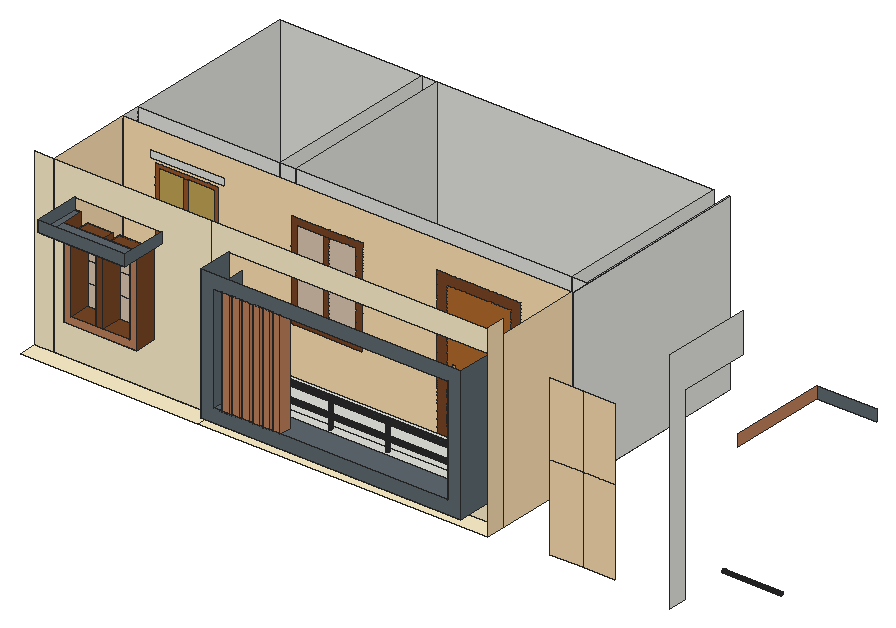
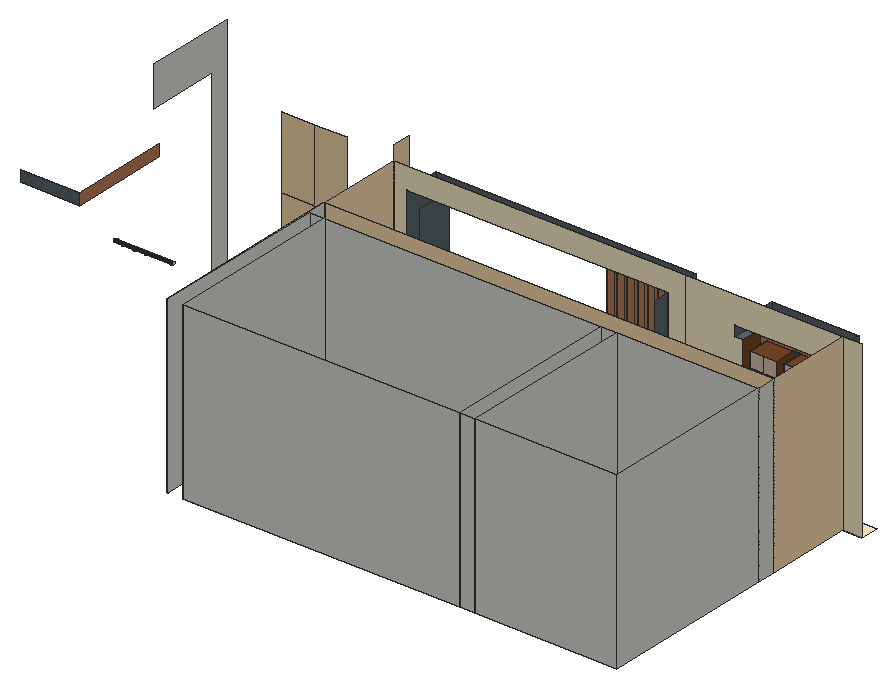
# SketchUp Ruby script. Lengths in inches.
U = 1.inch
M = Sketchup.active_model
def pt(a) = Geom::Point3d.new(a.map { |v| v * U })
def face(e, loops, mat)
  f = e.add_face(loops[0].map { |a| pt(a) })
  loops[1..].each { |l| e.add_face(l.map { |a| pt(a) }).erase! }
  f.material = f.back_material = mat if mat
  f
end
# faces: each face lists its corners as indices into pts; further lists are holes
def faces(e, pts, list, mat = nil) = list.each { |f| face(e, (f[0].is_a?(Array) ? f : [f]).map { |l| l.map { |i| pts[i] } }, mat) }
# xy, xz, yz: faces in a plane at the given z, y or x. An outline is a flat list of corners, or four numbers for a rectangle; further outlines are holes
def ring(l) = l.size == 4 ? [[l[0], l[1]], [l[2], l[1]], [l[2], l[3]], [l[0], l[3]]] : l.each_slice(2).to_a
def flat(e, list, mat, &to3) = list.each { |f| face(e, (f[0].is_a?(Array) ? f : [f]).map { |l| ring(l).map { |u, v| to3.(u, v) } }, mat) }
def xy(e, z, list, mat = nil) = flat(e, list, mat) { |x, y| [x, y, z] }
def xz(e, y, list, mat = nil) = flat(e, list, mat) { |x, z| [x, y, z] }
def yz(e, x, list, mat = nil) = flat(e, list, mat) { |y, z| [x, y, z] }
def lines(e, pts, list) = list.each { |a, b| e.add_line(pt(pts[a]), pt(pts[b])) }
# prism: a flat outline (further loops are holes) pulled along v
def prism(e, loops, v, mat = nil)
  f = face(e, loops, mat); d = Geom::Vector3d.new(v.map { |x| x * U })
  f.pushpull(f.normal.samedirection?(d) ? d.length : -d.length)
end
def box(e, o, s, mat = nil) = prism(e, [[o, [o[0] + s[0], o[1], o[2]], [o[0] + s[0], o[1] + s[1], o[2]], [o[0], o[1] + s[1], o[2]]]], [0, 0, s[2]], mat)
def at(x, y, z, deg = 0) = Geom::Transformation.translation(pt([x, y, z])) * Geom::Transformation.rotation(ORIGIN, Z_AXIS, deg.degrees)
def axes(o, x, y, z) = Geom::Transformation.new([*x, 0, *y, 0, *z, 0, *pt(o).to_a, 1])
def part(name) = M.definitions.add(name)
# library, detail: a bought-in or finely detailed component or shape, given as its bounding box
def library(name, o, s) = part(name).tap { |d| box(d.entities, o, s) }
def detail(e, o, s) = box(e.add_group.entities, o, s)
def put(e, d, t, mat = nil) = e.add_instance(d, t).tap { |i| i.material = mat if mat }
def group(e, t, mat = nil) = e.add_group.tap { |g| g.transformation = t; g.material = mat if mat }.entities
root = M.entities
M.materials.add("[Blinds Cloth Horizontal]").color = [192, 163, 85]
M.materials.add("[Color C01]").color = [221, 199, 177]
M.materials.add("[Color D01]").color = [255, 242, 204]
M.materials.add("[Formica Beige]").color = [255, 225, 180]
M.materials.add("[Formica Beige]1").color = [247, 219, 174]
M.materials.add("[Formica Laminate Dark]").color = [50, 53, 60]
M.materials.add("[Formica Speckled Grey]").color = [94, 105, 111]
M.materials.add("[Wood Bamboo]").color = [177, 105, 43]
M.materials.add("[Wood Cherry Original]").color = [152, 86, 42]
M.materials.add("[Wood Floor Light]").color = [204, 176, 127]
M.materials.add("[Wood Veneer 01]").color = [120, 70, 37]
M.materials.add("[Wood Veneer 02]").color = [190, 128, 91]
xy(root,536.125,[[47.7,166.1,1198.27,388.54],[47.7,388.54,1201.41,436.38],[1201.41,388.54,1201.79,436.38],[47.7,436.38,412.34,890.39],[412.34,436.38,451.3125,890.39],
  [451.3125,436.38,1159.05,890.39],[1198.27,436.38,1198.27,890.39,1201.41,436.38],[1201.41,436.38,1198.27,890.39,1201.41,890.39],[1201.41,436.38,1201.79,890.39]])
xy(root,536.125,[[0,119.17,455.68,166.1],[455.68,119.17,1198.27,166.1]],"[Color D01]")
xy(root,585.01,[[497.875,73.92,1164.39,166.1]],"[Formica Speckled Grey]")
xy(root,588.32,[[1811.85,227.29,1812.63,227.4,1813.35,227.69,1813.97,228.17,1814.45,228.79,1814.75,229.52,1814.85,230.29,1814.75,231.07,1814.45,231.79,1813.97,232.41,1813.35,232.89,1812.63,233.19,1811.85,233.29,1811.08,233.19,1810.35,232.89,1809.73,232.41,1809.25,231.79,1808.96,231.07,1808.85,230.29,1808.96,229.52,1809.25,228.79,1809.73,228.17,1810.35,227.69,1811.08,227.4]])
xy(root,588.82,[[1840.85,227.29,1841.63,227.4,1842.35,227.69,1842.97,228.17,1843.45,228.79,1843.75,229.52,1843.85,230.29,1843.75,231.07,1843.45,231.79,1842.97,232.41,1842.35,232.89,1841.63,233.19,1840.85,233.29,1840.08,233.19,1839.35,232.89,1838.73,232.41,1838.25,231.79,1837.96,231.07,1837.85,230.29,1837.96,229.52,1838.25,228.79,1838.73,228.17,1839.35,227.69,1840.08,227.4]])
xy(root,589.07,[[1780.92,227.29,1781.69,227.4,1782.42,227.69,1783.04,228.17,1783.51,228.79,1783.8125,229.52,1783.92,230.29,1783.8125,231.07,1783.51,231.79,1783.04,232.41,1782.42,232.89,1781.69,233.19,1780.92,233.29,1780.14,233.19,1779.42,232.89,1778.79,232.41,1778.32,231.79,1778.02,231.07,1777.92,230.29,1778.02,229.52,1778.32,228.79,1778.79,228.17,1779.42,227.69,1780.14,227.4]])
xy(root,591.76,[[1750.54,227.29,1751.32,227.4,1752.04,227.69,1752.66,228.17,1753.14,228.79,1753.4375,229.52,1753.54,230.29,1753.4375,231.07,1753.14,231.79,1752.66,232.41,1752.44,232.59,1748.65,232.59,1748.42,232.41,1747.94,231.79,1747.64,231.07,1747.54,230.29,1747.64,229.52,1747.94,228.79,1748.42,228.17,1749.04,227.69,1749.76,227.4],[1748.65,232.59,1752.44,232.59,1752.04,232.89,1751.32,233.19,1750.54,233.29,1749.76,233.19,1749.04,232.89]])
xy(root,592.19,[[1855.17,227.29,1855.94,227.4,1856.67,227.69,1857.29,228.17,1857.76,228.79,1858.0625,229.52,1858.17,230.29,1858.0625,231.07,1857.76,231.79,1857.29,232.41,1856.67,232.89,1855.94,233.19,1855.17,233.29,1854.39,233.19,1853.67,232.89,1853.04,232.41,1852.57,231.79,1852.27,231.07,1852.17,230.29,1852.27,229.52,1852.57,228.79,1853.04,228.17,1853.67,227.69,1854.39,227.4]])
xy(root,593.51,[[1722.85,227.29,1723.63,227.4,1724.35,227.69,1724.97,228.17,1725.45,228.79,1725.75,229.52,1725.85,230.29,1725.75,231.07,1725.45,231.79,1725.2,232.12,1720.5,232.12,1720.25,231.79,1719.96,231.07,1719.85,230.29,1719.96,229.52,1720.25,228.79,1720.73,228.17,1721.35,227.69,1722.08,227.4],[1720.5,232.12,1725.2,232.12,1724.97,232.41,1724.35,232.89,1723.63,233.19,1722.85,233.29,1722.08,233.19,1721.35,232.89,1720.73,232.41]])
xy(root,618.32,[[553.83,73.92,572.52,104.16],[579.27,73.92,597.96,104.16],[604.77,73.92,623.46,104.16],[631.58,73.92,650.27,104.16],[657.77,73.92,676.46,104.16],
  [683.15,73.92,701.83,104.16],[[531.18,142.13,1131.08,166.1],[617.04,150.12,616.01,150.25,615.04,150.65,614.22,151.29,613.58,152.12,613.18,153.08,613.04,154.12,613.18,155.15,613.58,156.12,614.22,156.95,615.04,157.58,616.01,157.98,617.04,158.12,618.08,157.98,619.04,157.58,619.87,156.95,620.51,156.12,620.91,155.15,621.04,154.12,620.91,153.08,620.51,152.12,619.87,151.29,619.04,150.65,618.08,150.25],[913.79,150.12,912.76,150.25,911.79,150.65,910.97,151.29,910.33,152.12,909.93,153.08,909.79,154.12,909.93,155.15,910.33,156.12,910.97,156.95,911.79,157.58,912.76,157.98,913.79,158.12,914.83,157.98,915.79,157.58,916.62,156.95,917.26,156.12,917.66,155.15,917.79,154.12,917.66,153.08,917.26,152.12,916.62,151.29,915.79,150.65,914.83,150.25],[767.42,150.12,766.38,150.25,765.42,150.65,764.59,151.29,763.95,152.12,763.56,153.08,763.42,154.12,763.56,155.15,763.95,156.12,764.59,156.95,765.42,157.58,766.38,157.98,767.42,158.12,768.45,157.98,769.42,157.58,770.25,156.95,770.88,156.12,771.28,155.15,771.42,154.12,771.28,153.08,770.88,152.12,770.25,151.29,769.42,150.65,768.45,150.25],[1075.98,150.12,1074.95,150.25,1073.98,150.65,1073.15,151.29,1072.52,152.12,1072.12,153.08,1071.98,154.12,1072.12,155.15,1072.52,156.12,1073.15,156.95,1073.98,157.58,1074.95,157.98,1075.98,158.12,1077.02,157.98,1077.98,157.58,1078.81,156.95,1079.45,156.12,1079.84,155.15,1079.98,154.12,1079.84,153.08,1079.45,152.12,1078.81,151.29,1077.98,150.65,1077.02,150.25]],[617.04,150.12,616.01,150.25,615.04,150.65,614.22,151.29,613.58,152.12,613.18,153.08,613.04,154.12,613.18,155.15,613.58,156.12,614.22,156.95,615.04,157.58,616.01,157.98,617.04,158.12,618.08,157.98,619.04,157.58,619.87,156.95,620.51,156.12,620.91,155.15,621.04,154.12,620.91,153.08,620.51,152.12,619.87,151.29,619.04,150.65,618.08,150.25],[767.42,150.12,766.38,150.25,765.42,150.65,764.59,151.29,763.95,152.12,763.56,153.08,763.42,154.12,763.56,155.15,763.95,156.12,764.59,156.95,765.42,157.58,766.38,157.98,767.42,158.12,768.45,157.98,769.42,157.58,770.25,156.95,770.88,156.12,771.28,155.15,771.42,154.12,771.28,153.08,770.88,152.12,770.25,151.29,769.42,150.65,768.45,150.25],[913.79,150.12,912.76,150.25,911.79,150.65,910.97,151.29,910.33,152.12,909.93,153.08,909.79,154.12,909.93,155.15,910.33,156.12,910.97,156.95,911.79,157.58,912.76,157.98,913.79,158.12,914.83,157.98,915.79,157.58,916.62,156.95,917.26,156.12,917.66,155.15,917.79,154.12,917.66,153.08,917.26,152.12,916.62,151.29,915.79,150.65,914.83,150.25],
  [1075.98,150.12,1074.95,150.25,1073.98,150.65,1073.15,151.29,1072.52,152.12,1072.12,153.08,1071.98,154.12,1072.12,155.15,1072.52,156.12,1073.15,156.95,1073.98,157.58,1074.95,157.98,1075.98,158.12,1077.02,157.98,1077.98,157.58,1078.81,156.95,1079.45,156.12,1079.84,155.15,1079.98,154.12,1079.84,153.08,1079.45,152.12,1078.81,151.29,1077.98,150.65,1077.02,150.25]])
xy(root,618.32,[[531.18,73.92,553.83,73.92,553.83,104.16,572.52,104.16,572.52,73.92,579.27,73.92,579.27,104.16,597.96,104.16,597.96,73.92,604.77,73.92,604.77,104.16,623.46,104.16,623.46,73.92,631.58,73.92,631.58,104.16,650.27,104.16,650.27,73.92,657.77,73.92,657.77,104.16,676.46,104.16,676.46,73.92,683.15,73.92,683.15,104.16,701.83,104.16,701.83,73.92,1131.08,73.92,1131.08,142.13,531.18,142.13]],"[Formica Speckled Grey]")
xy(root,654.42,[[117.05,111.6,304.55,166.1]],"[Wood Veneer 01]")
xy(root,672.82,[[135.45,111.6,199.22,166.1],[216.32,111.6,286.15,166.1]],"[Wood Veneer 01]")
xy(root,684.94,[[1075.98,150.12,1077.02,150.25,1077.98,150.65,1078.81,151.29,1079.45,152.12,1079.84,153.08,1079.98,154.12,1079.84,155.15,1079.45,156.12,1078.81,156.95,1077.98,157.58,1077.02,157.98,1075.98,158.12,1074.95,157.98,1073.98,157.58,1073.15,156.95,1072.52,156.12,1072.12,155.15,1071.98,154.12,1072.12,153.08,1072.52,152.12,1073.15,151.29,1073.98,150.65,1074.95,150.25]])
xy(root,686.94,[[913.79,150.12,914.83,150.25,915.79,150.65,916.62,151.29,917.26,152.12,917.66,153.08,917.79,154.12,917.66,155.15,917.26,156.12,916.62,156.95,915.79,157.58,914.83,157.98,913.79,158.12,912.76,157.98,911.79,157.58,910.97,156.95,910.33,156.12,909.93,155.15,909.79,154.12,909.93,153.08,910.33,152.12,910.97,151.29,911.79,150.65,912.76,150.25]])
xy(root,687.63,[[767.42,150.12,768.45,150.25,769.42,150.65,770.25,151.29,770.88,152.12,771.28,153.08,771.42,154.12,771.28,155.15,770.88,156.12,770.25,156.95,769.42,157.58,768.45,157.98,767.42,158.12,766.38,157.98,765.42,157.58,764.59,156.95,763.95,156.12,763.56,155.15,763.42,154.12,763.56,153.08,763.95,152.12,764.59,151.29,765.42,150.65,766.38,150.25]])
xy(root,688.88,[[617.04,150.12,618.08,150.25,619.04,150.65,619.87,151.29,620.51,152.12,620.91,153.08,621.04,154.12,620.91,155.15,620.51,156.12,619.87,156.95,619.04,157.58,618.08,157.98,617.04,158.12,616.01,157.98,615.04,157.58,614.22,156.95,613.58,156.12,613.18,155.15,613.04,154.12,613.18,153.08,613.58,152.12,614.22,151.29,615.04,150.65,616.01,150.25]])
xy(root,863.89,[[135.45,111.6,199.22,166.1],[216.32,111.6,286.15,166.1]],"[Wood Veneer 01]")
xy(root,882.3,[[100.99,47.54,117.05,166.1],[117.05,47.54,304.55,111.6],[304.55,47.54,326.11,166.1]],"[Formica Speckled Grey]")
xz(root,47.54,[[100.99,882.3,326.11,911.08]],"[Formica Speckled Grey]")
xz(root,73.92,[[[497.875,585.01,1164.39,925.7],[531.18,618.32,1131.08,892.39]]],"[Formica Speckled Grey]")
xz(root,73.92,[[553.83,618.32,572.52,892.39],[579.27,618.32,597.96,892.39],[604.77,618.32,623.46,892.39],[631.58,618.32,650.27,892.39],[657.77,618.32,676.46,892.39],
  [683.15,618.32,701.83,892.39]],"[Wood Veneer 02]")
xz(root,104.16,[[553.83,618.32,572.52,892.39],[579.27,618.32,597.96,892.39],[604.77,618.32,623.46,892.39],[631.58,618.32,650.27,892.39],[657.77,618.32,676.46,892.39],
  [683.15,618.32,701.83,892.39]],"[Wood Veneer 02]")
xz(root,111.6,[[199.22,672.82,216.32,863.89]],"[Wood Veneer 01]")
xz(root,111.6,[[[117.05,654.42,304.55,882.3],[135.45,672.82,286.15,863.89]]],"[Wood Veneer 02]")
xz(root,119.17,[[1358.02,552.78,1440.68,771.08],[1440.68,552.78,1523.35,771.08],[1358.02,771.08,1440.68,957.69],[1440.68,771.08,1523.35,957.69]],"[Formica Beige]1")
xz(root,166.1,[[135.45,672.82,167.34,726.34],[167.34,672.82,199.22,726.34],[216.32,672.82,251.23,726.34],[251.23,672.82,286.15,726.34],[135.45,726.34,167.34,779.86],
  [167.34,726.34,199.22,779.86],[216.32,726.34,251.23,779.86],[251.23,726.34,286.15,779.86],[135.45,779.86,167.34,824.51],[167.34,779.86,199.22,824.51],
  [216.32,779.86,251.23,824.51],[251.23,779.86,286.15,824.51],[135.45,824.51,167.34,863.89],[167.34,824.51,199.22,863.89],[216.32,824.51,251.23,863.89],
  [251.23,824.51,286.15,863.89]],"[Color C01]")
xz(root,166.1,[[0,536.125,47.7,980.9375],[[47.7,536.125,1198.27,980.3125],[497.875,585.01,1164.39,925.7],[117.05,654.42,117.05,882.3,100.99,882.3,100.99,911.08,326.11,911.08,326.11,882.3,304.55,882.3,304.55,654.42]]],"[Color D01]")
xz(root,388.54,[[1198.27,536.125,1201.41,980.3125],[1201.41,536.125,1201.79,980.3125]])
xz(root,388.54,[[142.36,701.45,201.48,892.8125],[216.65,701.45,279.66,892.8125]],"[Blinds Cloth Horizontal]")
xz(root,388.54,[[496.54,672.47,559.83,886.7],[575.8125,672.47,643.15,886.7]],"[Color C01]")
xz(root,388.54,[[[47.7,536.125,852.07,536.125,852.07,910.25,1068.07,910.25,1068.07,536.125,1198.27,536.125,1198.27,980.3125,47.7,980.3125],[477.9375,653.87,661.75,905.31],[130.08,689.16,291.95,905.1],[116.16,908.99,307.29,929.24]]],"[Formica Beige]")
xz(root,388.54,[[[877.66,561.71,1042.48,884.66],[890.09,623.15,901.34,708.15]]],"[Wood Bamboo]")
xz(root,388.54,[[[130.08,689.16,291.95,905.1],[142.36,701.45,279.66,892.8125]],[201.48,701.45,216.65,892.8125]],"[Wood Cherry Original]")
xz(root,388.54,[[890.09,623.15,901.34,708.15]],"[Wood Floor Light]")
xz(root,388.54,[[[852.07,536.125,1068.07,910.25],[877.66,561.71,1042.48,884.66]],[[477.9375,653.87,661.75,905.31],[496.54,672.47,643.15,886.7]],[559.83,672.47,575.8125,886.7]],"[Wood Veneer 01]")
xz(root,436.38,[[47.7,536.125,412.34,980.3125],[412.34,536.125,451.3125,980.3125],[451.3125,536.125,1159.05,980.3125],[1159.05,536.125,1198.27,980.3125]])
xz(root,528.45,[[1713.03,855.83,1866.15,885.01]],"[Formica Speckled Grey]")
xz(root,890.39,[[47.7,536.125,412.34,980.9375],[412.34,536.125,451.3125,980.9375],[451.3125,536.125,1159.05,980.9375],[1198.27,536.125,1201.41,980.3125],[1201.41,536.125,1201.79,536.125,1201.79,980.9375,1198.27,980.9375,1198.27,980.3125,1201.41,980.3125]])
yz(root,47.7,[[388.54,536.125,436.38,980.3125],[436.38,536.125,890.39,980.9375]])
yz(root,47.7,[[166.1,536.125,388.54,980.9375]],"[Formica Beige]")
yz(root,100.99,[[47.54,882.3,166.1,911.08]],"[Formica Speckled Grey]")
yz(root,117.05,[[111.6,654.42,166.1,882.3]],"[Wood Veneer 01]")
yz(root,135.45,[[111.6,672.82,166.1,863.89]],"[Wood Veneer 01]")
yz(root,199.22,[[111.6,672.82,166.1,863.89]],"[Wood Veneer 01]")
yz(root,216.32,[[111.6,672.82,166.1,863.89]],"[Wood Veneer 01]")
yz(root,286.15,[[111.6,672.82,166.1,863.89]],"[Wood Veneer 01]")
yz(root,304.55,[[111.6,654.42,166.1,882.3]],"[Wood Veneer 01]")
yz(root,326.11,[[47.54,882.3,166.1,911.08]],"[Formica Speckled Grey]")
yz(root,412.34,[[436.38,536.125,890.39,980.9375]])
yz(root,451.3125,[[436.38,536.125,890.39,980.9375]])
yz(root,497.875,[[73.92,585.01,166.1,925.7]],"[Formica Speckled Grey]")
yz(root,531.18,[[[73.92,618.32,166.1,892.39],[154.12,682.76,152.55,682.96,151.09,683.57,149.83,684.53,148.87,685.79,148.26,687.25,148.05,688.82,148.26,690.39,148.87,691.85,149.83,693.11,151.09,694.07,152.55,694.68,154.12,694.88,155.6875,694.68,157.15,694.07,158.4,693.11,159.37,691.85,159.97,690.39,160.18,688.82,159.97,687.25,159.37,685.79,158.4,684.53,157.15,683.57,155.6875,682.96],[154.12,643.43,152.69,643.62,151.37,644.17,150.23,645.04,149.35,646.18,148.8,647.51,148.62,648.93,148.8,650.36,149.35,651.68,150.23,652.82,151.37,653.7,152.69,654.25,154.12,654.43,155.54,654.25,156.87,653.7,158.01,652.82,158.88,651.68,159.43,650.36,159.62,648.93,159.43,647.51,158.88,646.18,158.01,645.04,156.87,644.17,155.54,643.62]]],"[Formica Speckled Grey]")
yz(root,553.83,[[73.92,618.32,104.16,892.39]],"[Wood Veneer 02]")
yz(root,572.52,[[73.92,618.32,104.16,892.39]],"[Wood Veneer 02]")
yz(root,579.27,[[73.92,618.32,104.16,892.39]],"[Wood Veneer 02]")
yz(root,597.96,[[73.92,618.32,104.16,892.39]],"[Wood Veneer 02]")
yz(root,604.77,[[73.92,618.32,104.16,892.39]],"[Wood Veneer 02]")
yz(root,623.46,[[73.92,618.32,104.16,892.39]],"[Wood Veneer 02]")
yz(root,631.58,[[73.92,618.32,104.16,892.39]],"[Wood Veneer 02]")
yz(root,650.27,[[73.92,618.32,104.16,892.39]],"[Wood Veneer 02]")
yz(root,657.77,[[73.92,618.32,104.16,892.39]],"[Wood Veneer 02]")
yz(root,676.46,[[73.92,618.32,104.16,892.39]],"[Wood Veneer 02]")
yz(root,683.15,[[73.92,618.32,104.16,892.39]],"[Wood Veneer 02]")
yz(root,701.83,[[73.92,618.32,104.16,892.39]],"[Wood Veneer 02]")
yz(root,1131.08,[[154.12,643.43,155.54,643.62,156.87,644.17,158.01,645.04,158.88,646.18,159.43,647.51,159.62,648.93,159.43,650.36,158.88,651.68,158.01,652.82,156.87,653.7,155.54,654.25,154.12,654.43,152.69,654.25,151.37,653.7,150.23,652.82,149.35,651.68,148.8,650.36,148.62,648.93,148.8,647.51,149.35,646.18,150.23,645.04,151.37,644.17,152.69,643.62],[154.12,682.76,155.6875,682.96,157.15,683.57,158.4,684.53,159.37,685.79,159.97,687.25,160.18,688.82,159.97,690.39,159.37,691.85,158.4,693.11,157.15,694.07,155.6875,694.68,154.12,694.88,152.55,694.68,151.09,694.07,149.83,693.11,148.87,691.85,148.26,690.39,148.05,688.82,148.26,687.25,148.87,685.79,149.83,684.53,151.09,683.57,152.55,682.96]])
yz(root,1131.08,[[[73.92,618.32,166.1,892.39],[154.12,682.76,155.6875,682.96,157.15,683.57,158.4,684.53,159.37,685.79,159.97,687.25,160.18,688.82,159.97,690.39,159.37,691.85,158.4,693.11,157.15,694.07,155.6875,694.68,154.12,694.88,152.55,694.68,151.09,694.07,149.83,693.11,148.87,691.85,148.26,690.39,148.05,688.82,148.26,687.25,148.87,685.79,149.83,684.53,151.09,683.57,152.55,682.96],[154.12,643.43,155.54,643.62,156.87,644.17,158.01,645.04,158.88,646.18,159.43,647.51,159.62,648.93,159.43,650.36,158.88,651.68,158.01,652.82,156.87,653.7,155.54,654.25,154.12,654.43,152.69,654.25,151.37,653.7,150.23,652.82,149.35,651.68,148.8,650.36,148.62,648.93,148.8,647.51,149.35,646.18,150.23,645.04,151.37,644.17,152.69,643.62]]],"[Formica Speckled Grey]")
yz(root,1159.05,[[436.38,536.125,890.39,980.9375]])
yz(root,1164.39,[[73.92,585.01,166.1,925.7]],"[Formica Speckled Grey]")
yz(root,1198.27,[[436.38,536.125,890.39,980.3125]])
yz(root,1198.27,[[166.1,536.125,388.54,980.3125]],"[Formica Beige]")
yz(root,1198.27,[[119.17,536.125,119.17,1016.9375,166.04,1016.9375,166.04,980.3125,166.1,980.3125,166.1,536.125]],"[Formica Beige]1")
yz(root,1201.41,[[388.54,536.125,890.39,980.3125]])
yz(root,1201.79,[[388.54,536.125,890.39,980.3125]])
yz(root,1665.33,[[119.17,536.125,166.04,536.125,166.04,1016.9375,351.29,1016.9375,351.29,1119.0625,119.17,1119.0625]])
yz(root,1713.03,[[229.09,588.26,228.18,588.375,227.34,588.73,226.61,589.28,226.06,590.01,225.71,590.85,225.59,591.76,225.71,592.66,226.06,593.51,226.61,594.23,227.34,594.79,228.18,595.14,229.09,595.26,229.99,595.14,230.84,594.79,231.5625,594.23,232.12,593.51,232.47,592.66,232.59,591.76,232.47,590.85,232.12,590.01,231.5625,589.28,230.84,588.73,229.99,588.375]])
yz(root,1713.03,[[274.61,855.83,528.45,885.01]],"[Wood Veneer 02]")
yz(root,1863.4,[[229.09,588.26,229.99,588.375,230.84,588.73,231.5625,589.28,232.12,590.01,232.47,590.85,232.59,591.76,232.47,592.66,232.12,593.51,231.5625,594.23,230.84,594.79,229.99,595.14,229.09,595.26,228.18,595.14,227.34,594.79,226.61,594.23,226.06,593.51,225.71,592.66,225.59,591.76,225.71,590.85,226.06,590.01,226.61,589.28,227.34,588.73,228.18,588.375]],"[Formica Laminate Dark]")
p = [[1713.03,228.18,588.375],[1713.03,229.09,588.26],[1863.4,229.09,588.26],[1863.4,228.18,588.375],[1713.03,229.99,588.375],[1863.4,229.99,588.375],
  [1713.03,227.34,588.73],[1863.4,227.34,588.73],[1713.03,230.84,588.73],[1863.4,230.84,588.73],[1713.03,226.61,589.28],[1863.4,226.61,589.28],
  [1713.03,231.5625,589.28],[1863.4,231.5625,589.28],[1713.03,226.06,590.01],[1863.4,226.06,590.01],[1713.03,232.12,590.01],[1863.4,232.12,590.01],
  [1713.03,225.71,590.85],[1863.4,225.71,590.85],[1713.03,232.47,590.85],[1863.4,232.47,590.85],[1713.03,225.59,591.76],[1863.4,225.59,591.76],
  [1713.03,232.59,591.76],[1748.65,232.59,591.76],[1752.44,232.59,591.76],[1863.4,232.59,591.76],[1713.03,225.71,592.66],[1863.4,225.71,592.66],
  [1713.03,232.47,592.66],[1863.4,232.47,592.66],[1713.03,226.06,593.51],[1863.4,226.06,593.51],[1713.03,232.12,593.51],[1720.5,232.12,593.51],
  [1725.2,232.12,593.51],[1863.4,232.12,593.51],[1713.03,226.61,594.23],[1863.4,226.61,594.23],[1713.03,231.5625,594.23],[1863.4,231.5625,594.23],
  [1713.03,227.34,594.79],[1863.4,227.34,594.79],[1713.03,230.84,594.79],[1863.4,230.84,594.79],[1713.03,228.18,595.14],[1863.4,228.18,595.14],
  [1713.03,229.99,595.14],[1863.4,229.99,595.14],[1713.03,229.09,595.26],[1863.4,229.09,595.26],[616.01,150.25,618.32],[617.04,150.12,618.32],
  [617.04,150.12,688.88],[616.01,150.25,688.88],[618.08,150.25,618.32],[618.08,150.25,688.88],[766.38,150.25,618.32],[767.42,150.12,618.32],
  [767.42,150.12,687.63],[766.38,150.25,687.63],[768.45,150.25,618.32],[768.45,150.25,687.63],[912.76,150.25,618.32],[913.79,150.12,618.32],
  [913.79,150.12,686.94],[912.76,150.25,686.94],[914.83,150.25,618.32],[914.83,150.25,686.94],[1074.95,150.25,618.32],[1075.98,150.12,618.32],
  [1075.98,150.12,684.94],[1074.95,150.25,684.94],[1077.02,150.25,618.32],[1077.02,150.25,684.94],[615.04,150.65,618.32],[615.04,150.65,688.88],
  [619.04,150.65,618.32],[619.04,150.65,688.88],[765.42,150.65,618.32],[765.42,150.65,687.63],[769.42,150.65,618.32],[769.42,150.65,687.63],
  [911.79,150.65,618.32],[911.79,150.65,686.94],[915.79,150.65,618.32],[915.79,150.65,686.94],[1073.98,150.65,618.32],[1073.98,150.65,684.94],
  [1077.98,150.65,618.32],[1077.98,150.65,684.94],[614.22,151.29,618.32],[614.22,151.29,688.88],[619.87,151.29,618.32],[619.87,151.29,688.88],
  [764.59,151.29,618.32],[764.59,151.29,687.63],[770.25,151.29,618.32],[770.25,151.29,687.63],[910.97,151.29,618.32],[910.97,151.29,686.94],
  [916.62,151.29,618.32],[916.62,151.29,686.94],[1073.15,151.29,618.32],[1073.15,151.29,684.94],[1078.81,151.29,618.32],[1078.81,151.29,684.94],
  [613.58,152.12,618.32],[613.58,152.12,688.88],[620.51,152.12,618.32],[620.51,152.12,688.88],[763.95,152.12,618.32],[763.95,152.12,687.63],
  [770.88,152.12,618.32],[770.88,152.12,687.63],[910.33,152.12,618.32],[910.33,152.12,686.94],[917.26,152.12,618.32],[917.26,152.12,686.94],
  [1072.52,152.12,618.32],[1072.52,152.12,684.94],[1079.45,152.12,618.32],[1079.45,152.12,684.94],[613.18,153.08,618.32],[613.18,153.08,688.88],
  [620.91,153.08,618.32],[620.91,153.08,688.88],[763.56,153.08,618.32],[763.56,153.08,687.63],[771.28,153.08,618.32],[771.28,153.08,687.63],
  [909.93,153.08,618.32],[909.93,153.08,686.94],[917.66,153.08,618.32],[917.66,153.08,686.94],[1072.12,153.08,618.32],[1072.12,153.08,684.94],
  [1079.84,153.08,618.32],[1079.84,153.08,684.94],[613.04,154.12,618.32],[613.04,154.12,688.88],[613.04,154.12,682.76],[613.04,154.12,654.43],
  [613.04,154.12,643.43],[621.04,154.12,618.32],[621.04,154.12,643.43],[621.04,154.12,654.43],[621.04,154.12,682.76],[621.04,154.12,688.88],
  [763.42,154.12,618.32],[763.42,154.12,687.63],[763.42,154.12,682.76],[763.42,154.12,654.43],[763.42,154.12,643.43],[771.42,154.12,618.32],
  [771.42,154.12,643.43],[771.42,154.12,654.43],[771.42,154.12,682.76],[771.42,154.12,687.63],[909.79,154.12,618.32],[909.79,154.12,686.94],
  [909.79,154.12,682.76],[909.79,154.12,654.43],[909.79,154.12,643.43],[917.79,154.12,618.32],[917.79,154.12,643.43],[917.79,154.12,654.43],
  [917.79,154.12,682.76],[917.79,154.12,686.94],[1071.98,154.12,618.32],[1071.98,154.12,684.94],[1071.98,154.12,682.76],[1071.98,154.12,654.43],
  [1071.98,154.12,643.43],[1079.98,154.12,618.32],[1079.98,154.12,643.43],[1079.98,154.12,654.43],[1079.98,154.12,682.76],[1079.98,154.12,684.94],
  [613.18,155.15,618.32],[613.18,155.15,688.88],[620.91,155.15,618.32],[620.91,155.15,688.88],[763.56,155.15,618.32],[763.56,155.15,687.63],
  [771.28,155.15,618.32],[771.28,155.15,687.63],[909.93,155.15,618.32],[909.93,155.15,686.94],[917.66,155.15,618.32],[917.66,155.15,686.94],
  [1072.12,155.15,618.32],[1072.12,155.15,684.94],[1079.84,155.15,618.32],[1079.84,155.15,684.94],[613.58,156.12,618.32],[613.58,156.12,688.88],
  [620.51,156.12,618.32],[620.51,156.12,688.88],[763.95,156.12,618.32],[763.95,156.12,687.63],[770.88,156.12,618.32],[770.88,156.12,687.63],
  [910.33,156.12,618.32],[910.33,156.12,686.94],[917.26,156.12,618.32],[917.26,156.12,686.94],[1072.52,156.12,618.32],[1072.52,156.12,684.94],
  [1079.45,156.12,618.32],[1079.45,156.12,684.94],[614.22,156.95,618.32],[614.22,156.95,688.88],[619.87,156.95,618.32],[619.87,156.95,688.88],
  [764.59,156.95,618.32],[764.59,156.95,687.63],[770.25,156.95,618.32],[770.25,156.95,687.63],[910.97,156.95,618.32],[910.97,156.95,686.94],
  [916.62,156.95,618.32],[916.62,156.95,686.94],[1073.15,156.95,618.32],[1073.15,156.95,684.94],[1078.81,156.95,618.32],[1078.81,156.95,684.94],
  [615.04,157.58,618.32],[615.04,157.58,688.88],[619.04,157.58,618.32],[619.04,157.58,688.88],[765.42,157.58,618.32],[765.42,157.58,687.63],
  [769.42,157.58,618.32],[769.42,157.58,687.63],[911.79,157.58,618.32],[911.79,157.58,686.94],[915.79,157.58,618.32],[915.79,157.58,686.94],
  [1073.98,157.58,618.32],[1073.98,157.58,684.94],[1077.98,157.58,618.32],[1077.98,157.58,684.94],[616.01,157.98,618.32],[616.01,157.98,688.88],
  [618.08,157.98,618.32],[618.08,157.98,688.88],[766.38,157.98,618.32],[766.38,157.98,687.63],[768.45,157.98,618.32],[768.45,157.98,687.63],
  [912.76,157.98,618.32],[912.76,157.98,686.94],[914.83,157.98,618.32],[914.83,157.98,686.94],[1074.95,157.98,618.32],[1074.95,157.98,684.94],
  [1077.02,157.98,618.32],[1077.02,157.98,684.94],[617.04,158.12,618.32],[617.04,158.12,688.88],[767.42,158.12,618.32],[767.42,158.12,687.63],
  [913.79,158.12,618.32],[913.79,158.12,686.94],[1075.98,158.12,618.32],[1075.98,158.12,684.94],[1131.08,154.12,643.43],[1131.08,152.69,643.62],
  [531.18,152.69,643.62],[531.18,154.12,643.43],[1131.08,155.54,643.62],[531.18,155.54,643.62],[1131.08,151.37,644.17],[531.18,151.37,644.17],
  [1131.08,156.87,644.17],[531.18,156.87,644.17],[1131.08,150.23,645.04],[531.18,150.23,645.04],[1131.08,158.01,645.04],[531.18,158.01,645.04],
  [1131.08,149.35,646.18],[531.18,149.35,646.18],[1131.08,158.88,646.18],[531.18,158.88,646.18],[1131.08,148.8,647.51],[531.18,148.8,647.51],
  [1131.08,159.43,647.51],[531.18,159.43,647.51],[1131.08,148.62,648.93],[531.18,148.62,648.93],[1131.08,159.62,648.93],[531.18,159.62,648.93],
  [1131.08,148.8,650.36],[531.18,148.8,650.36],[1131.08,159.43,650.36],[531.18,159.43,650.36],[1131.08,149.35,651.68],[531.18,149.35,651.68],
  [1131.08,158.88,651.68],[531.18,158.88,651.68],[1131.08,150.23,652.82],[531.18,150.23,652.82],[1131.08,158.01,652.82],[531.18,158.01,652.82],
  [1131.08,151.37,653.7],[531.18,151.37,653.7],[1131.08,156.87,653.7],[531.18,156.87,653.7],[1131.08,152.69,654.25],[531.18,152.69,654.25],
  [1131.08,155.54,654.25],[531.18,155.54,654.25],[1131.08,154.12,654.43],[531.18,154.12,654.43],[1131.08,154.12,682.76],[1131.08,152.55,682.96],
  [531.18,152.55,682.96],[531.18,154.12,682.76],[1131.08,155.6875,682.96],[531.18,155.6875,682.96],[1131.08,151.09,683.57],[531.18,151.09,683.57],
  [1131.08,157.15,683.57],[531.18,157.15,683.57],[1131.08,149.83,684.53],[531.18,149.83,684.53],[1131.08,158.4,684.53],[531.18,158.4,684.53],
  [1131.08,148.87,685.79],[531.18,148.87,685.79],[1131.08,159.37,685.79],[531.18,159.37,685.79],[1131.08,148.26,687.25],[531.18,148.26,687.25],
  [1131.08,159.97,687.25],[531.18,159.97,687.25],[1131.08,148.05,688.82],[531.18,148.05,688.82],[1131.08,160.18,688.82],[531.18,160.18,688.82],
  [1131.08,148.26,690.39],[531.18,148.26,690.39],[1131.08,159.97,690.39],[531.18,159.97,690.39],[1131.08,148.87,691.85],[531.18,148.87,691.85],
  [1131.08,159.37,691.85],[531.18,159.37,691.85],[1131.08,149.83,693.11],[531.18,149.83,693.11],[1131.08,158.4,693.11],[531.18,158.4,693.11],
  [1131.08,151.09,694.07],[531.18,151.09,694.07],[1131.08,157.15,694.07],[531.18,157.15,694.07],[1131.08,152.55,694.68],[531.18,152.55,694.68],
  [1131.08,155.6875,694.68],[531.18,155.6875,694.68],[1131.08,154.12,694.88],[531.18,154.12,694.88],[455.68,166.1,536.125],[451.36,166.08,980.3125]]
faces(root,p,[[0,1,2,3],[1,4,5,2],[6,0,3,7],[4,8,9,5],[10,6,7,11],[8,12,13,9],[14,10,11,15],[12,16,17,13],
  [18,14,15,19],[16,20,21,17],[22,18,19,23],[20,24,25,26,27,21],[28,22,23,29],[24,30,31,27,26,25],[32,28,29,33],[30,34,35,36,37,31],
  [38,32,33,39],[34,40,41,37,36,35],[42,38,39,43],[40,44,45,41],[46,42,43,47],[44,48,49,45],[50,46,47,51],[48,50,51,49],
  [52,53,54,55],[53,56,57,54],[58,59,60,61],[59,62,63,60],[64,65,66,67],[65,68,69,66],[70,71,72,73],[71,74,75,72],
  [76,52,55,77],[56,78,79,57],[80,58,61,81],[62,82,83,63],[84,64,67,85],[68,86,87,69],[88,70,73,89],[74,90,91,75],
  [92,76,77,93],[78,94,95,79],[96,80,81,97],[82,98,99,83],[100,84,85,101],[86,102,103,87],[104,88,89,105],[90,106,107,91],
  [108,92,93,109],[94,110,111,95],[112,96,97,113],[98,114,115,99],[116,100,101,117],[102,118,119,103],[120,104,105,121],[106,122,123,107],
  [124,108,109,125],[110,126,127,111],[128,112,113,129],[114,130,131,115],[132,116,117,133],[118,134,135,119],[136,120,121,137],[122,138,139,123],
  [140,124,125,141,142,143,144],[126,145,146,147,148,149,127],[150,128,129,151,152,153,154],[130,155,156,157,158,159,131],[160,132,133,161,162,163,164],[134,165,166,167,168,169,135],[170,136,137,171,172,173,174],[138,175,176,177,178,179,139],
  [180,140,144,143,142,141,181],[145,182,183,149,148,147,146],[184,150,154,153,152,151,185],[155,186,187,159,158,157,156],[188,160,164,163,162,161,189],[165,190,191,169,168,167,166],[192,170,174,173,172,171,193],[175,194,195,179,178,177,176],
  [196,180,181,197],[182,198,199,183],[200,184,185,201],[186,202,203,187],[204,188,189,205],[190,206,207,191],[208,192,193,209],[194,210,211,195],
  [212,196,197,213],[198,214,215,199],[216,200,201,217],[202,218,219,203],[220,204,205,221],[206,222,223,207],[224,208,209,225],[210,226,227,211],
  [228,212,213,229],[214,230,231,215],[232,216,217,233],[218,234,235,219],[236,220,221,237],[222,238,239,223],[240,224,225,241],[226,242,243,227],
  [244,228,229,245],[230,246,247,231],[248,232,233,249],[234,250,251,235],[252,236,237,253],[238,254,255,239],[256,240,241,257],[242,258,259,243],
  [260,244,245,261],[246,260,261,247],[262,248,249,263],[250,262,263,251],[264,252,253,265],[254,264,265,255],[266,256,257,267],[258,266,267,259],
  [268,269,270,271,144,146,154,156,164,166,174,176],[272,268,176,174,166,164,156,154,146,144,271,273],[269,274,275,270],[276,272,273,277],[274,278,279,275],[280,276,277,281],[278,282,283,279],[284,280,281,285],
  [282,286,287,283],[288,284,285,289],[286,290,291,287],[292,288,289,293],[290,294,295,291],[296,292,293,297],[294,298,299,295],[300,296,297,301],
  [298,302,303,299],[304,300,301,305],[302,306,307,303],[308,304,305,309],[306,310,311,307],[312,308,309,313],[310,314,177,173,167,163,157,153,147,143,315,311],[314,312,313,315,143,147,153,157,163,167,173,177],
  [316,317,318,319,142,148,152,158,162,168,172,178],[320,316,178,172,168,162,158,152,148,142,319,321],[317,322,323,318],[324,320,321,325],[322,326,327,323],[328,324,325,329],[326,330,331,327],[332,328,329,333],
  [330,334,335,331],[336,332,333,337],[334,338,339,335],[340,336,337,341],[338,342,343,339],[344,340,341,345],[342,346,347,343],[348,344,345,349],
  [346,350,351,347],[352,348,349,353],[350,354,355,351],[356,352,353,357],[354,358,359,355],[360,356,357,361],[358,362,363,359],[362,360,361,363]],"[Formica Laminate Dark]")
lines(root,p,[[364,365]])
